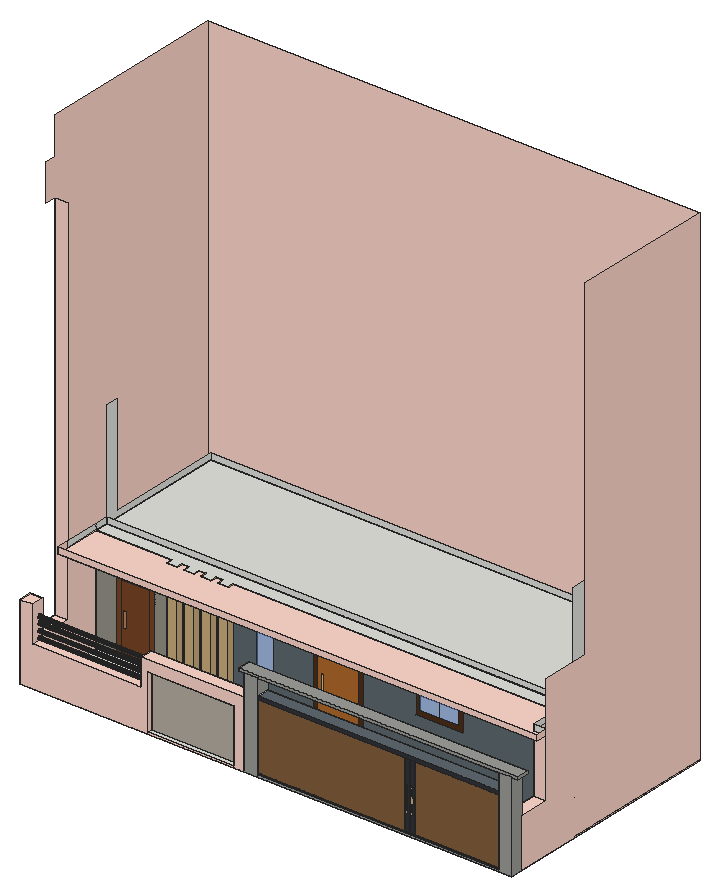
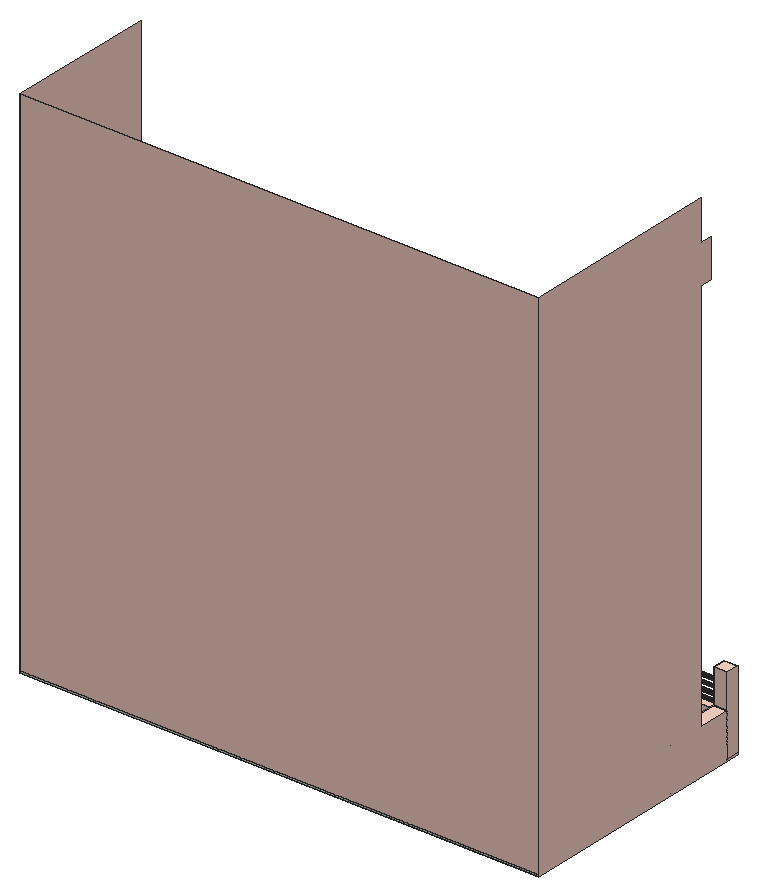
# SketchUp Ruby script. Lengths in inches.
U = 1.inch
M = Sketchup.active_model
def pt(a) = Geom::Point3d.new(a.map { |v| v * U })
def face(e, loops, mat)
  f = e.add_face(loops[0].map { |a| pt(a) })
  loops[1..].each { |l| e.add_face(l.map { |a| pt(a) }).erase! }
  f.material = f.back_material = mat if mat
  f
end
# faces: each face lists its corners as indices into pts; further lists are holes
def faces(e, pts, list, mat = nil) = list.each { |f| face(e, (f[0].is_a?(Array) ? f : [f]).map { |l| l.map { |i| pts[i] } }, mat) }
# xy, xz, yz: faces in a plane at the given z, y or x. An outline is a flat list of corners, or four numbers for a rectangle; further outlines are holes
def ring(l) = l.size == 4 ? [[l[0], l[1]], [l[2], l[1]], [l[2], l[3]], [l[0], l[3]]] : l.each_slice(2).to_a
def flat(e, list, mat, &to3) = list.each { |f| face(e, (f[0].is_a?(Array) ? f : [f]).map { |l| ring(l).map { |u, v| to3.(u, v) } }, mat) }
def xy(e, z, list, mat = nil) = flat(e, list, mat) { |x, y| [x, y, z] }
def xz(e, y, list, mat = nil) = flat(e, list, mat) { |x, z| [x, y, z] }
def yz(e, x, list, mat = nil) = flat(e, list, mat) { |y, z| [x, y, z] }
def lines(e, pts, list) = list.each { |a, b| e.add_line(pt(pts[a]), pt(pts[b])) }
# prism: a flat outline (further loops are holes) pulled along v
def prism(e, loops, v, mat = nil)
  f = face(e, loops, mat); d = Geom::Vector3d.new(v.map { |x| x * U })
  f.pushpull(f.normal.samedirection?(d) ? d.length : -d.length)
end
def box(e, o, s, mat = nil) = prism(e, [[o, [o[0] + s[0], o[1], o[2]], [o[0] + s[0], o[1] + s[1], o[2]], [o[0], o[1] + s[1], o[2]]]], [0, 0, s[2]], mat)
def at(x, y, z, deg = 0) = Geom::Transformation.translation(pt([x, y, z])) * Geom::Transformation.rotation(ORIGIN, Z_AXIS, deg.degrees)
def axes(o, x, y, z) = Geom::Transformation.new([*x, 0, *y, 0, *z, 0, *pt(o).to_a, 1])
def part(name) = M.definitions.add(name)
# library, detail: a bought-in or finely detailed component or shape, given as its bounding box
def library(name, o, s) = part(name).tap { |d| box(d.entities, o, s) }
def detail(e, o, s) = box(e.add_group.entities, o, s)
def put(e, d, t, mat = nil) = e.add_instance(d, t).tap { |i| i.material = mat if mat }
def group(e, t, mat = nil) = e.add_group.tap { |g| g.transformation = t; g.material = mat if mat }.entities
root = M.entities
M.materials.add("[Blinds Wood Bamboo]").color = [131, 94, 60]
M.materials.add("[Color B01]").color = [255, 216, 204]
M.materials.add("[Concrete Block 8x8 Gray]").color = [157, 158, 154]
M.materials.add("[Concrete Block 8x8 Gray]1").color = [157, 158, 154]
M.materials.add("[Formica Graystone]").color = [149, 146, 135]
M.materials.add("[Formica Laminate Dark]").color = [50, 53, 60]
M.materials.add("[Formica Speckled Grey]").color = [94, 105, 111]
M.materials.add("[Stone Masonry Multi]").color = [182, 175, 164]
M.materials.add("[Translucent Glass Blue]").color = [100, 149, 237]
M.materials["[Translucent Glass Blue]"].alpha = 0.5
M.materials.add("[Wood Bamboo]").color = [177, 105, 43]
M.materials.add("[Wood Floor Light]").color = [204, 176, 127]
M.materials.add("[Wood OSB]").color = [240, 195, 122]
M.materials.add("[Wood Veneer 01]").color = [79, 46, 24]
M.materials.add("[Wood Veneer 01]1").color = [120, 70, 37]
M.materials.add("[Wood Veneer 02]").color = [190, 128, 91]
xy(root,0,[[0,0,3040.15,1455.17]])
xy(root,9,[[0,0,77.93,77.93],[791.24,0,1324.84,31.9375],[1324.84,0,1383.6875,77.93],[1470.93,0,2962.22,77.93],[791.24,31.9375,1324.84,77.93],
  [77.93,77.93,2962.22,77.93,2962.22,488.625,927.87,488.625,927.87,450.4375,863.29,450.4375,863.29,488.625,821.87,488.625,821.87,450.4375,757.29,450.4375,757.29,488.625,716.43,488.625,716.43,450.4375,651.86,450.4375,651.86,488.625,611.18,488.625,611.18,450.4375,546.61,450.4375,546.61,488.625,77.93,488.625],[77.93,571.9,2962.22,1377.24]])
xy(root,14.52,[[1470.93,0,2962.22,77.93]])
xy(root,21.81,[[1470.93,0,2383.51,77.93],[2383.51,0,2412.92,77.93],[2412.92,0,2442.33,77.93],[2442.33,0,2962.22,77.93]])
xy(root,245.9375,[[77.93,0,748.1,77.93]],"[Color B01]")
xy(root,266.0625,[[0,77.93,77.93,267.5625]],"[Color B01]")
xy(root,300.8125,[[2962.22,77.93,3040.15,267.5625]],"[Color B01]")
xy(root,344.47,[[791.24,0,1324.84,31.9375]])
xy(root,411.875,[[748.1,0,1383.6875,77.93]],"[Color B01]")
xy(root,427.16,[[2412.92,0,2442.33,77.93]])
xy(root,447.93,[[1470.93,0,2962.22,77.93]],"[Formica Speckled Grey]")
xy(root,467.75,[[0,0,77.93,77.93]],"[Color B01]")
xy(root,549.125,[[1355.84,0,1383.6875,77.93],[1383.6875,0,1470.93,77.93],[2962.22,0,3040.15,77.93],[3040.15,0,3081.84,77.93]])
xy(root,549.125,[[1470.93,0,2962.22,77.93]],"[Concrete Block 8x8 Gray]")
xy(root,565.5625,[[1355.84,0,3081.84,77.93]],"[Concrete Block 8x8 Gray]")
xy(root,664.1875,[[546.61,450.4375,546.61,488.625,77.93,488.625,77.93,571.9,2962.22,571.9,2962.22,488.625,927.87,488.625,927.87,450.4375,863.29,450.4375,863.29,488.625,821.87,488.625,821.87,450.4375,757.29,450.4375,757.29,488.625,716.43,488.625,716.43,450.4375,651.86,450.4375,651.86,488.625,611.18,488.625,611.18,450.4375],[77.93,571.9,2962.22,1377.24]])
xy(root,664.1875,[[77.93,195.0625,77.93,488.625,546.61,488.625,546.61,450.4375,611.18,450.4375,611.18,488.625,651.86,488.625,651.86,450.4375,716.43,450.4375,716.43,488.625,757.29,488.625,757.29,450.4375,821.87,450.4375,821.87,488.625,863.29,488.625,863.29,450.4375,927.87,450.4375,927.87,488.625,2962.22,488.625,2962.22,267.5625,3040.15,267.5625,3040.15,195.0625]],"[Color B01]")
xz(root,0,[[1470.93,21.81,2383.51,427.16],[2442.33,21.81,2962.22,427.16]],"[Blinds Wood Bamboo]")
xz(root,0,[[0,0,1383.6875,0,1383.6875,9,791.24,9,791.24,344.47,1324.84,344.47,1324.84,9,1383.6875,9,1383.6875,411.875,748.1,411.875,748.1,245.9375,77.93,245.9375,77.93,467.75,0,467.75]],"[Color B01]")
xz(root,0,[[1383.6875,0,3040.15,0,3040.15,549.125,2962.22,549.125,2962.22,9,1470.93,9,1470.93,549.125,1383.6875,549.125],[1355.84,549.125,3081.84,565.5625]],"[Concrete Block 8x8 Gray]")
xz(root,0,[[1470.93,14.52,2962.22,21.81],[[2383.51,21.81,2412.92,427.16],[2389.22,124.65,2401.4,286.59]],[[2412.92,21.81,2442.33,427.16],[2420.22,124.65,2432.4,286.59]],[1470.93,427.16,2962.22,447.93]],"[Formica Laminate Dark]")
xz(root,0,[[2389.22,124.65,2401.4,286.59],[2420.22,124.65,2432.4,286.59]],"[Wood Floor Light]")
xz(root,31.9375,[[791.24,9,1324.84,344.47]],"[Stone Masonry Multi]")
xz(root,77.93,[[0,9,77.93,266.0625],[748.1,9,791.24,344.47],[1383.6875,9,1470.93,549.125],[1470.93,14.52,2962.22,21.81],[2383.51,21.81,2412.92,427.16],
  [2412.92,21.81,2442.33,427.16]])
xz(root,77.93,[[77.93,9,748.1,245.9375],[1324.84,9,1324.84,344.47,748.1,344.47,748.1,411.875,1383.6875,411.875,1383.6875,9],[791.24,9,1324.84,344.47],[0,266.0625,77.93,467.75]],"[Color B01]")
xz(root,77.93,[[1355.84,549.125,3081.84,565.5625]],"[Concrete Block 8x8 Gray]")
xz(root,77.93,[[2962.22,300.8125,3040.15,549.125]],"[Concrete Block 8x8 Gray]1")
xz(root,77.93,[[1470.93,21.81,2383.51,427.16],[2442.33,21.81,2962.22,427.16],[1470.93,427.16,2962.22,447.93]],"[Formica Speckled Grey]")
xz(root,195.0625,[[77.93,664.1875,3040.15,700.1875]],"[Color B01]")
xz(root,267.5625,[[2962.22,664.1875,3040.15,700.1875]])
xz(root,267.5625,[[0,266.0625,77.93,2577.9375],[2962.22,300.8125,3040.15,664.1875]],"[Color B01]")
xz(root,450.4375,[[546.61,9,611.18,664.1875],[651.86,9,716.43,664.1875],[757.29,9,821.87,664.1875],[863.29,9,927.87,664.1875]],"[Wood Floor Light]")
xz(root,488.625,[[77.93,9,200.99,9,200.99,481.125,444.24,481.125,444.24,9,546.61,9,546.61,664.1875,77.93,664.1875],[611.18,9,651.86,664.1875],[716.43,9,757.29,664.1875],[821.87,9,863.29,664.1875]],"[Formica Graystone]")
xz(root,488.625,[[[927.87,9,1419.05,9,1419.05,568.25,1733.67,568.25,1733.67,9,2962.22,9,2962.22,664.1875,927.87,664.1875],[2055.67,336.59,2352.77,583.45],[1075.93,237.42,1177.62,502.55]]],"[Formica Speckled Grey]")
xz(root,488.625,[[1075.93,237.42,1177.62,502.55],[2085.24,366.16,2204.22,460.02],[2204.22,366.16,2323.21,460.02],[2085.24,460.02,2204.22,553.88],[2204.22,460.02,2323.21,553.88]],"[Translucent Glass Blue]")
xz(root,488.625,[[[1452.16,42.11,1700.5625,535.14],[1468.27,235.88,1489.08,363.19]]],"[Wood Bamboo]")
xz(root,488.625,[[1468.27,235.88,1489.08,363.19]],"[Wood OSB]")
xz(root,488.625,[[[1419.05,9,1733.67,568.25],[1452.16,42.11,1700.5625,535.14]],[[2055.67,336.59,2352.77,583.45],[2085.24,366.16,2323.21,553.88]]],"[Wood Veneer 01]")
xz(root,488.625,[[[200.99,9,444.24,481.125],[232.57,40.57,412.67,449.55]],[[232.57,40.57,412.67,449.55],[250.67,181.08,264.17,276.39]]],"[Wood Veneer 01]1")
xz(root,488.625,[[250.67,181.08,264.17,276.39]],"[Wood Veneer 02]")
xz(root,571.9,[[77.93,9,2962.22,664.1875],[77.93,664.1875,2962.22,700.1875]])
xz(root,1377.24,[[77.93,9,2962.22,664.1875],[77.93,664.1875,2962.22,700.1875]])
xz(root,1455.17,[[0,0,3040.15,9]])
xz(root,1455.17,[[0,9,3040.15,3039.125]],"[Color B01]")
yz(root,0,[[0,0,0,9,77.93,9,77.93,266.0625,267.5625,266.0625,267.5625,2577.9375,195.0625,2577.9375,195.0625,2806.5,267.5625,2806.5,267.5625,3039.125,1455.17,3039.125,1455.17,0],[0,9,77.93,467.75]],"[Color B01]")
yz(root,77.93,[[488.625,9,571.9,664.1875],[571.9,9,1377.24,664.1875],[267.5625,664.1875,488.625,700.1875],[488.625,664.1875,571.9,700.1875],[571.9,664.1875,571.9,1321.0625,653.97,1321.0625,653.97,700.1875,1377.24,700.1875,1377.24,664.1875]])
yz(root,77.93,[[77.93,9,488.625,9,488.625,664.1875,267.5625,664.1875,267.5625,266.0625,77.93,266.0625],[[0,245.9375,77.93,467.75],[43.13,374.79,40.79,375.1,38.6,376,36.73,377.44,35.28,379.32,34.38,381.51,34.07,383.85,34.38,386.2,35.28,388.38,36.73,390.26,38.6,391.7,40.79,392.61,43.13,392.92,45.48,392.61,47.66,391.7,49.54,390.26,50.98,388.38,51.89,386.2,52.2,383.85,51.89,381.51,50.98,379.32,49.54,377.44,47.66,376,45.48,375.1],[44.45,336.92,42.1,337.22,39.92,338.13,38.04,339.57,36.6,341.45,35.7,343.63,35.39,345.98,35.7,348.32,36.6,350.51,38.04,352.39,39.92,353.83,42.1,354.73,44.45,355.04,46.8,354.73,48.98,353.83,50.86,352.39,52.3,350.51,53.2,348.32,53.51,345.98,53.2,343.63,52.3,341.45,50.86,339.57,48.98,338.13,46.8,337.22],[43.13,296.1,40.79,296.41,38.6,297.32,36.73,298.76,35.28,300.63,34.38,302.82,34.07,305.17,34.38,307.51,35.28,309.7,36.73,311.57,38.6,313.01,40.79,313.92,43.13,314.23,45.48,313.92,47.66,313.01,49.54,311.57,50.98,309.7,51.89,307.51,52.2,305.17,51.89,302.82,50.98,300.63,49.54,298.76,47.66,297.32,45.48,296.41],[43.13,257.17,40.79,257.47,38.6,258.38,36.73,259.82,35.28,261.7,34.38,263.88,34.07,266.23,34.38,268.57,35.28,270.76,36.73,272.64,38.6,274.08,40.79,274.98,43.13,275.29,45.48,274.98,47.66,274.08,49.54,272.64,50.98,270.76,51.89,268.57,52.2,266.23,51.89,263.88,50.98,261.7,49.54,259.82,47.66,258.38,45.48,257.47]],[195.0625,664.1875,267.5625,700.1875]],"[Color B01]")
yz(root,546.61,[[450.4375,9,488.625,664.1875]],"[Wood Floor Light]")
yz(root,611.18,[[450.4375,9,488.625,664.1875]],"[Wood Floor Light]")
yz(root,651.86,[[450.4375,9,488.625,664.1875]],"[Wood Floor Light]")
yz(root,716.43,[[450.4375,9,488.625,664.1875]],"[Wood Floor Light]")
yz(root,748.1,[[43.13,257.17,45.48,257.47,47.66,258.38,49.54,259.82,50.98,261.7,51.89,263.88,52.2,266.23,51.89,268.57,50.98,270.76,49.54,272.64,47.66,274.08,45.48,274.98,43.13,275.29,40.79,274.98,38.6,274.08,36.73,272.64,35.28,270.76,34.38,268.57,34.07,266.23,34.38,263.88,35.28,261.7,36.73,259.82,38.6,258.38,40.79,257.47],[43.13,296.1,45.48,296.41,47.66,297.32,49.54,298.76,50.98,300.63,51.89,302.82,52.2,305.17,51.89,307.51,50.98,309.7,49.54,311.57,47.66,313.01,45.48,313.92,43.13,314.23,40.79,313.92,38.6,313.01,36.73,311.57,35.28,309.7,34.38,307.51,34.07,305.17,34.38,302.82,35.28,300.63,36.73,298.76,38.6,297.32,40.79,296.41],[44.45,336.92,46.8,337.22,48.98,338.13,50.86,339.57,52.3,341.45,53.2,343.63,53.51,345.98,53.2,348.32,52.3,350.51,50.86,352.39,48.98,353.83,46.8,354.73,44.45,355.04,42.1,354.73,39.92,353.83,38.04,352.39,36.6,350.51,35.7,348.32,35.39,345.98,35.7,343.63,36.6,341.45,38.04,339.57,39.92,338.13,42.1,337.22],[43.13,374.79,45.48,375.1,47.66,376,49.54,377.44,50.98,379.32,51.89,381.51,52.2,383.85,51.89,386.2,50.98,388.38,49.54,390.26,47.66,391.7,45.48,392.61,43.13,392.92,40.79,392.61,38.6,391.7,36.73,390.26,35.28,388.38,34.38,386.2,34.07,383.85,34.38,381.51,35.28,379.32,36.73,377.44,38.6,376,40.79,375.1]])
yz(root,748.1,[[[0,245.9375,77.93,411.875],[43.13,374.79,45.48,375.1,47.66,376,49.54,377.44,50.98,379.32,51.89,381.51,52.2,383.85,51.89,386.2,50.98,388.38,49.54,390.26,47.66,391.7,45.48,392.61,43.13,392.92,40.79,392.61,38.6,391.7,36.73,390.26,35.28,388.38,34.38,386.2,34.07,383.85,34.38,381.51,35.28,379.32,36.73,377.44,38.6,376,40.79,375.1],[43.13,257.17,45.48,257.47,47.66,258.38,49.54,259.82,50.98,261.7,51.89,263.88,52.2,266.23,51.89,268.57,50.98,270.76,49.54,272.64,47.66,274.08,45.48,274.98,43.13,275.29,40.79,274.98,38.6,274.08,36.73,272.64,35.28,270.76,34.38,268.57,34.07,266.23,34.38,263.88,35.28,261.7,36.73,259.82,38.6,258.38,40.79,257.47],[44.45,336.92,46.8,337.22,48.98,338.13,50.86,339.57,52.3,341.45,53.2,343.63,53.51,345.98,53.2,348.32,52.3,350.51,50.86,352.39,48.98,353.83,46.8,354.73,44.45,355.04,42.1,354.73,39.92,353.83,38.04,352.39,36.6,350.51,35.7,348.32,35.39,345.98,35.7,343.63,36.6,341.45,38.04,339.57,39.92,338.13,42.1,337.22],[43.13,296.1,45.48,296.41,47.66,297.32,49.54,298.76,50.98,300.63,51.89,302.82,52.2,305.17,51.89,307.51,50.98,309.7,49.54,311.57,47.66,313.01,45.48,313.92,43.13,314.23,40.79,313.92,38.6,313.01,36.73,311.57,35.28,309.7,34.38,307.51,34.07,305.17,34.38,302.82,35.28,300.63,36.73,298.76,38.6,297.32,40.79,296.41]]],"[Color B01]")
yz(root,757.29,[[450.4375,9,488.625,664.1875]],"[Wood Floor Light]")
yz(root,791.24,[[31.9375,9,77.93,344.47]])
yz(root,791.24,[[0,9,31.9375,344.47]],"[Color B01]")
yz(root,821.87,[[450.4375,9,488.625,664.1875]],"[Wood Floor Light]")
yz(root,863.29,[[450.4375,9,488.625,664.1875]],"[Wood Floor Light]")
yz(root,927.87,[[450.4375,9,488.625,664.1875]],"[Wood Floor Light]")
yz(root,1324.84,[[31.9375,9,77.93,344.47]])
yz(root,1324.84,[[0,9,31.9375,344.47]],"[Color B01]")
yz(root,1355.84,[[0,549.125,77.93,565.5625]],"[Concrete Block 8x8 Gray]")
yz(root,1383.6875,[[0,9,77.93,411.875]])
yz(root,1383.6875,[[0,411.875,77.93,549.125]],"[Concrete Block 8x8 Gray]1")
yz(root,1470.93,[[0,9,77.93,14.52],[0,14.52,77.93,21.81],[0,21.81,77.93,427.16],[0,427.16,77.93,447.93]])
yz(root,1470.93,[[0,447.93,77.93,549.125]],"[Concrete Block 8x8 Gray]")
yz(root,2383.51,[[0,21.81,77.93,427.16]])
yz(root,2412.92,[[0,21.81,77.93,427.16]])
yz(root,2442.33,[[0,21.81,77.93,427.16]])
yz(root,2962.22,[[0,9,77.93,14.52],[488.625,9,571.9,664.1875],[571.9,9,1377.24,664.1875],[0,14.52,77.93,21.81],[0,21.81,77.93,427.16],
  [0,427.16,77.93,447.93],[267.5625,664.1875,488.625,700.1875],[488.625,664.1875,571.9,700.1875],[571.9,664.1875,1377.24,664.1875,1377.24,700.1875,653.97,700.1875,653.97,1321.0625,571.9,1321.0625]])
yz(root,2962.22,[[77.93,9,77.93,300.8125,267.5625,300.8125,267.5625,664.1875,488.625,664.1875,488.625,9]],"[Color B01]")
yz(root,2962.22,[[0,447.93,77.93,549.125]],"[Concrete Block 8x8 Gray]")
yz(root,3040.15,[[77.93,0,1455.17,0,1455.17,3039.125,571.9,3039.125,571.9,976.6875,267.5625,976.6875,267.5625,300.8125,77.93,300.8125],[195.0625,664.1875,267.5625,700.1875]],"[Color B01]")
yz(root,3040.15,[[0,0,77.93,549.125]],"[Concrete Block 8x8 Gray]1")
yz(root,3081.84,[[0,549.125,77.93,565.5625]],"[Concrete Block 8x8 Gray]")
p = [[748.1,43.13,257.17],[748.1,40.79,257.47],[77.93,40.79,257.47],[77.93,43.13,257.17],[748.1,45.48,257.47],[77.93,45.48,257.47],
  [748.1,38.6,258.38],[77.93,38.6,258.38],[748.1,47.66,258.38],[77.93,47.66,258.38],[748.1,36.73,259.82],[77.93,36.73,259.82],
  [748.1,49.54,259.82],[77.93,49.54,259.82],[748.1,35.28,261.7],[77.93,35.28,261.7],[748.1,50.98,261.7],[77.93,50.98,261.7],
  [748.1,34.38,263.88],[77.93,34.38,263.88],[748.1,51.89,263.88],[77.93,51.89,263.88],[748.1,34.07,266.23],[77.93,34.07,266.23],
  [748.1,52.2,266.23],[77.93,52.2,266.23],[748.1,34.38,268.57],[77.93,34.38,268.57],[748.1,51.89,268.57],[77.93,51.89,268.57],
  [748.1,35.28,270.76],[77.93,35.28,270.76],[748.1,50.98,270.76],[77.93,50.98,270.76],[748.1,36.73,272.64],[77.93,36.73,272.64],
  [748.1,49.54,272.64],[77.93,49.54,272.64],[748.1,38.6,274.08],[77.93,38.6,274.08],[748.1,47.66,274.08],[77.93,47.66,274.08],
  [748.1,40.79,274.98],[77.93,40.79,274.98],[748.1,45.48,274.98],[77.93,45.48,274.98],[748.1,43.13,275.29],[77.93,43.13,275.29],
  [748.1,43.13,296.1],[748.1,40.79,296.41],[77.93,40.79,296.41],[77.93,43.13,296.1],[748.1,45.48,296.41],[77.93,45.48,296.41],
  [748.1,38.6,297.32],[77.93,38.6,297.32],[748.1,47.66,297.32],[77.93,47.66,297.32],[748.1,36.73,298.76],[77.93,36.73,298.76],
  [748.1,49.54,298.76],[77.93,49.54,298.76],[748.1,35.28,300.63],[77.93,35.28,300.63],[748.1,50.98,300.63],[77.93,50.98,300.63],
  [748.1,34.38,302.82],[77.93,34.38,302.82],[748.1,51.89,302.82],[77.93,51.89,302.82],[748.1,34.07,305.17],[77.93,34.07,305.17],
  [748.1,52.2,305.17],[77.93,52.2,305.17],[748.1,34.38,307.51],[77.93,34.38,307.51],[748.1,51.89,307.51],[77.93,51.89,307.51],
  [748.1,35.28,309.7],[77.93,35.28,309.7],[748.1,50.98,309.7],[77.93,50.98,309.7],[748.1,36.73,311.57],[77.93,36.73,311.57],
  [748.1,49.54,311.57],[77.93,49.54,311.57],[748.1,38.6,313.01],[77.93,38.6,313.01],[748.1,47.66,313.01],[77.93,47.66,313.01],
  [748.1,40.79,313.92],[77.93,40.79,313.92],[748.1,45.48,313.92],[77.93,45.48,313.92],[748.1,43.13,314.23],[77.93,43.13,314.23],
  [748.1,44.45,336.92],[748.1,42.1,337.22],[77.93,42.1,337.22],[77.93,44.45,336.92],[748.1,46.8,337.22],[77.93,46.8,337.22],
  [748.1,39.92,338.13],[77.93,39.92,338.13],[748.1,48.98,338.13],[77.93,48.98,338.13],[748.1,38.04,339.57],[77.93,38.04,339.57],
  [748.1,50.86,339.57],[77.93,50.86,339.57],[748.1,36.6,341.45],[77.93,36.6,341.45],[748.1,52.3,341.45],[77.93,52.3,341.45],
  [748.1,35.7,343.63],[77.93,35.7,343.63],[748.1,53.2,343.63],[77.93,53.2,343.63],[748.1,35.39,345.98],[77.93,35.39,345.98],
  [748.1,53.51,345.98],[77.93,53.51,345.98],[748.1,35.7,348.32],[77.93,35.7,348.32],[748.1,53.2,348.32],[77.93,53.2,348.32],
  [748.1,36.6,350.51],[77.93,36.6,350.51],[748.1,52.3,350.51],[77.93,52.3,350.51],[748.1,38.04,352.39],[77.93,38.04,352.39],
  [748.1,50.86,352.39],[77.93,50.86,352.39],[748.1,39.92,353.83],[77.93,39.92,353.83],[748.1,48.98,353.83],[77.93,48.98,353.83],
  [748.1,42.1,354.73],[77.93,42.1,354.73],[748.1,46.8,354.73],[77.93,46.8,354.73],[748.1,44.45,355.04],[77.93,44.45,355.04],
  [748.1,43.13,374.79],[748.1,40.79,375.1],[77.93,40.79,375.1],[77.93,43.13,374.79],[748.1,45.48,375.1],[77.93,45.48,375.1],
  [748.1,38.6,376],[77.93,38.6,376],[748.1,47.66,376],[77.93,47.66,376],[748.1,36.73,377.44],[77.93,36.73,377.44],
  [748.1,49.54,377.44],[77.93,49.54,377.44],[748.1,35.28,379.32],[77.93,35.28,379.32],[748.1,50.98,379.32],[77.93,50.98,379.32],
  [748.1,34.38,381.51],[77.93,34.38,381.51],[748.1,51.89,381.51],[77.93,51.89,381.51],[748.1,34.07,383.85],[77.93,34.07,383.85],
  [748.1,52.2,383.85],[77.93,52.2,383.85],[748.1,34.38,386.2],[77.93,34.38,386.2],[748.1,51.89,386.2],[77.93,51.89,386.2],
  [748.1,35.28,388.38],[77.93,35.28,388.38],[748.1,50.98,388.38],[77.93,50.98,388.38],[748.1,36.73,390.26],[77.93,36.73,390.26],
  [748.1,49.54,390.26],[77.93,49.54,390.26],[748.1,38.6,391.7],[77.93,38.6,391.7],[748.1,47.66,391.7],[77.93,47.66,391.7],
  [748.1,40.79,392.61],[77.93,40.79,392.61],[748.1,45.48,392.61],[77.93,45.48,392.61],[748.1,43.13,392.92],[77.93,43.13,392.92],
  [3040.15,488.625,9],[3040.15,1455.17,9],[0,488.625,9],[77.93,488.625,9],[2962.22,488.625,9],[2962.22,488.625,226.1875],
  [3040.15,488.625,226.1875],[0,488.625,266.0625],[77.93,488.625,266.0625]]
faces(root,p,[[0,1,2,3],[4,0,3,5],[1,6,7,2],[8,4,5,9],[6,10,11,7],[12,8,9,13],[10,14,15,11],[16,12,13,17],
  [14,18,19,15],[20,16,17,21],[18,22,23,19],[24,20,21,25],[22,26,27,23],[28,24,25,29],[26,30,31,27],[32,28,29,33],
  [30,34,35,31],[36,32,33,37],[34,38,39,35],[40,36,37,41],[38,42,43,39],[44,40,41,45],[42,46,47,43],[46,44,45,47],
  [48,49,50,51],[52,48,51,53],[49,54,55,50],[56,52,53,57],[54,58,59,55],[60,56,57,61],[58,62,63,59],[64,60,61,65],
  [62,66,67,63],[68,64,65,69],[66,70,71,67],[72,68,69,73],[70,74,75,71],[76,72,73,77],[74,78,79,75],[80,76,77,81],
  [78,82,83,79],[84,80,81,85],[82,86,87,83],[88,84,85,89],[86,90,91,87],[92,88,89,93],[90,94,95,91],[94,92,93,95],
  [96,97,98,99],[100,96,99,101],[97,102,103,98],[104,100,101,105],[102,106,107,103],[108,104,105,109],[106,110,111,107],[112,108,109,113],
  [110,114,115,111],[116,112,113,117],[114,118,119,115],[120,116,117,121],[118,122,123,119],[124,120,121,125],[122,126,127,123],[128,124,125,129],
  [126,130,131,127],[132,128,129,133],[130,134,135,131],[136,132,133,137],[134,138,139,135],[140,136,137,141],[138,142,143,139],[142,140,141,143],
  [144,145,146,147],[148,144,147,149],[145,150,151,146],[152,148,149,153],[150,154,155,151],[156,152,153,157],[154,158,159,155],[160,156,157,161],
  [158,162,163,159],[164,160,161,165],[162,166,167,163],[168,164,165,169],[166,170,171,167],[172,168,169,173],[170,174,175,171],[176,172,173,177],
  [174,178,179,175],[180,176,177,181],[178,182,183,179],[184,180,181,185],[182,186,187,183],[188,184,185,189],[186,190,191,187],[190,188,189,191]],"[Wood Veneer 02]")
lines(root,p,[[192,193],[194,195],[196,192],[197,198],[199,200]])
